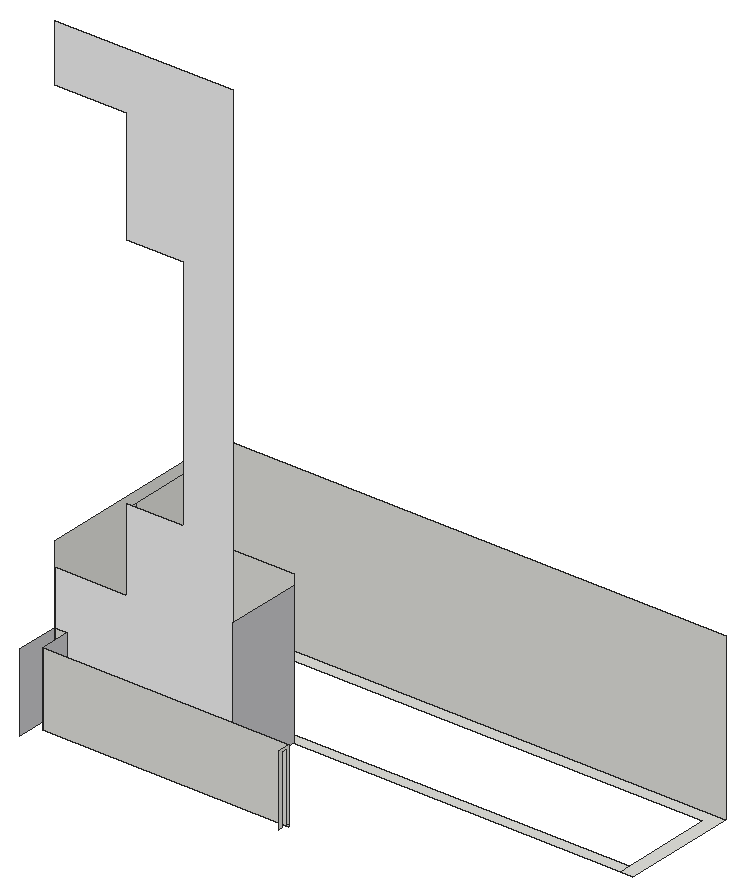
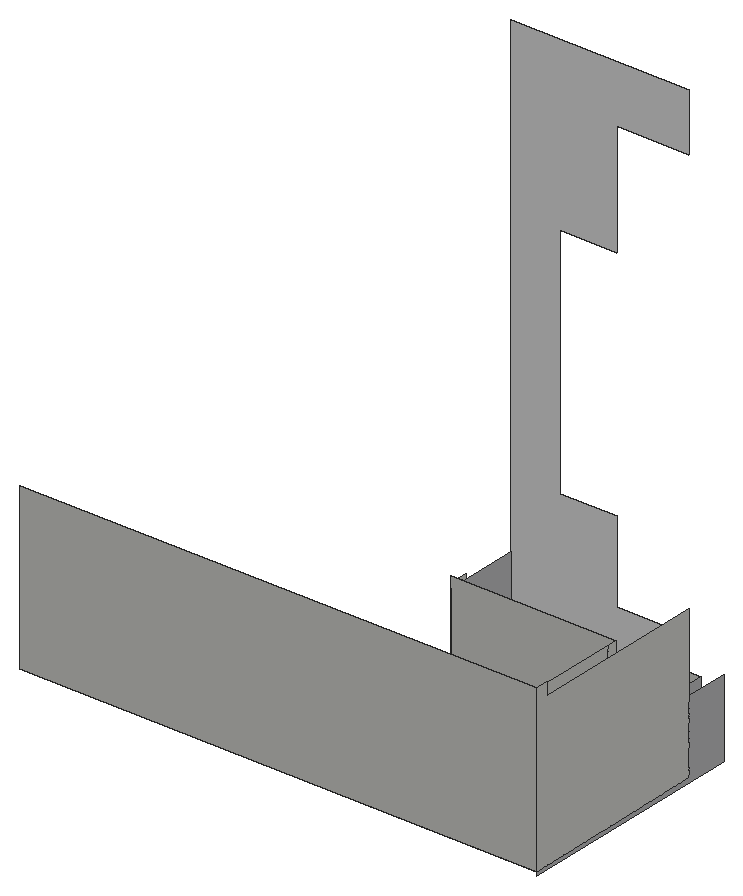
# SketchUp Ruby script. Lengths in inches.
U = 1.inch
M = Sketchup.active_model
def pt(a) = Geom::Point3d.new(a.map { |v| v * U })
def face(e, loops, mat)
  f = e.add_face(loops[0].map { |a| pt(a) })
  loops[1..].each { |l| e.add_face(l.map { |a| pt(a) }).erase! }
  f.material = f.back_material = mat if mat
  f
end
# faces: each face lists its corners as indices into pts; further lists are holes
def faces(e, pts, list, mat = nil) = list.each { |f| face(e, (f[0].is_a?(Array) ? f : [f]).map { |l| l.map { |i| pts[i] } }, mat) }
# xy, xz, yz: faces in a plane at the given z, y or x. An outline is a flat list of corners, or four numbers for a rectangle; further outlines are holes
def ring(l) = l.size == 4 ? [[l[0], l[1]], [l[2], l[1]], [l[2], l[3]], [l[0], l[3]]] : l.each_slice(2).to_a
def flat(e, list, mat, &to3) = list.each { |f| face(e, (f[0].is_a?(Array) ? f : [f]).map { |l| ring(l).map { |u, v| to3.(u, v) } }, mat) }
def xy(e, z, list, mat = nil) = flat(e, list, mat) { |x, y| [x, y, z] }
def xz(e, y, list, mat = nil) = flat(e, list, mat) { |x, z| [x, y, z] }
def yz(e, x, list, mat = nil) = flat(e, list, mat) { |y, z| [x, y, z] }
def lines(e, pts, list) = list.each { |a, b| e.add_line(pt(pts[a]), pt(pts[b])) }
# prism: a flat outline (further loops are holes) pulled along v
def prism(e, loops, v, mat = nil)
  f = face(e, loops, mat); d = Geom::Vector3d.new(v.map { |x| x * U })
  f.pushpull(f.normal.samedirection?(d) ? d.length : -d.length)
end
def box(e, o, s, mat = nil) = prism(e, [[o, [o[0] + s[0], o[1], o[2]], [o[0] + s[0], o[1] + s[1], o[2]], [o[0], o[1] + s[1], o[2]]]], [0, 0, s[2]], mat)
def at(x, y, z, deg = 0) = Geom::Transformation.translation(pt([x, y, z])) * Geom::Transformation.rotation(ORIGIN, Z_AXIS, deg.degrees)
def axes(o, x, y, z) = Geom::Transformation.new([*x, 0, *y, 0, *z, 0, *pt(o).to_a, 1])
def part(name) = M.definitions.add(name)
# library, detail: a bought-in or finely detailed component or shape, given as its bounding box
def library(name, o, s) = part(name).tap { |d| box(d.entities, o, s) }
def detail(e, o, s) = box(e.add_group.entities, o, s)
def put(e, d, t, mat = nil) = e.add_instance(d, t).tap { |i| i.material = mat if mat }
def group(e, t, mat = nil) = e.add_group.tap { |g| g.transformation = t; g.material = mat if mat }.entities
root = M.entities
M.materials.add("[Cladding Siding White]").color = [242, 242, 242]
M.materials.add("[Polished Concrete New]").color = [200, 200, 203]
xy(root,9,[[11.875,314.12,11.875,714.96,1099.23,714.96,1099.23,472.99,1072.84,472.99,1072.84,688.57,38.27,688.57,38.27,314.12],[38.27,314.12,386.67,472.99],[38.27,472.99,1072.84,494.96]])
xz(root,249.9,[[38.27,9,555.05,163.5625]])
xz(root,314.12,[[11.875,9,38.27,163.5625]])
xz(root,314.12,[[38.27,9,386.67,9,386.67,1306.5625,11.875,1306.5625,11.875,1185.41,163.125,1185.41,163.125,947.1,282.875,947.1,282.875,450.91,163.125,450.91,163.125,278.16,11.875,278.16,11.875,163.5625,38.27,163.5625]],"[Cladding Siding White]")
xz(root,472.99,[[38.27,9,386.67,328.125]])
xz(root,714.96,[[11.875,9,1099.23,354.875]])
yz(root,11.875,[[314.12,9,314.12,328.125,688.57,328.125,688.57,354.875,714.96,354.875,714.96,9]])
yz(root,11.875,[[223.5,0,223.5,163.5625,314.12,163.5625,314.12,9,714.96,9,714.96,0]],"[Polished Concrete New]")
yz(root,38.27,[[472.99,9,494.96,328.125],[494.96,9,688.57,328.125]])
yz(root,38.27,[[249.9,9,314.12,163.5625]],"[Polished Concrete New]")
yz(root,386.67,[[314.12,9,472.99,304.3125]],"[Polished Concrete New]")
yz(root,555.05,[[223.5,14.9375,230.47,14.9375,230.47,158.26,244.05,158.26,244.05,14.9375,249.9,14.9375,249.9,163.5625,223.5,163.5625]])
